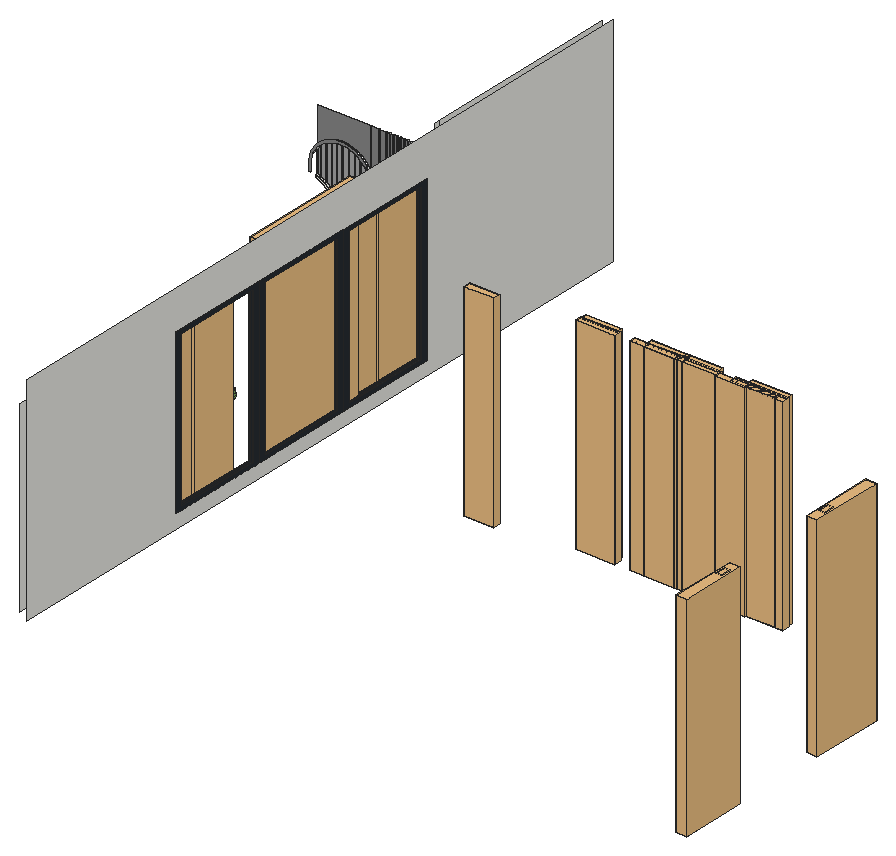
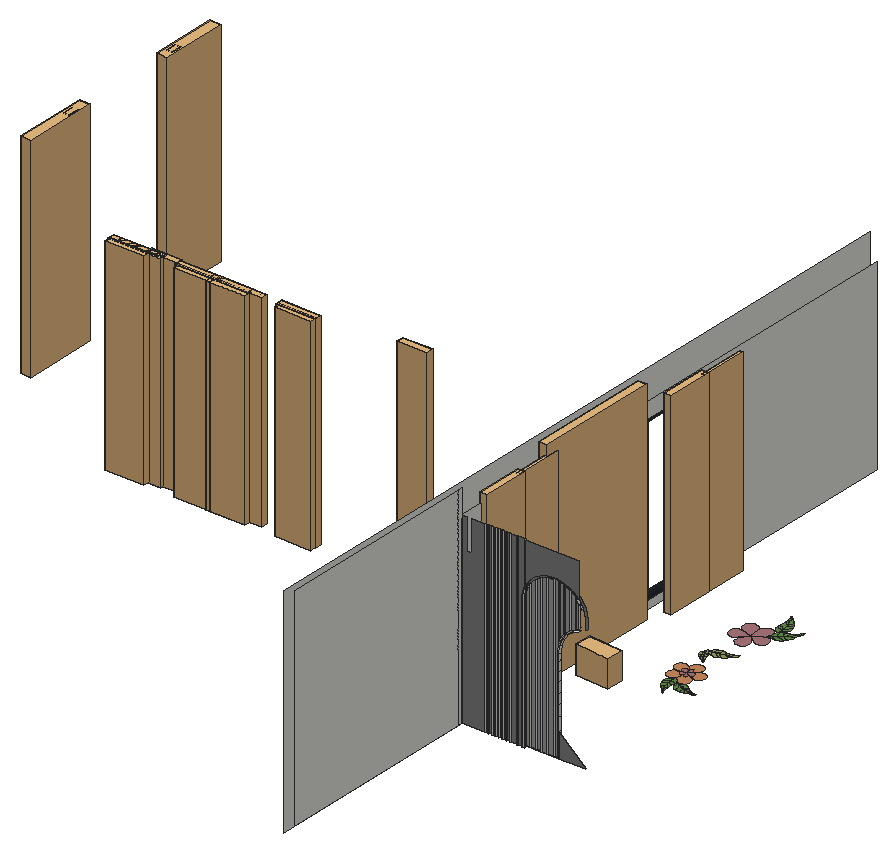
# SketchUp Ruby script. Lengths in inches.
U = 1.inch
M = Sketchup.active_model
def pt(a) = Geom::Point3d.new(a.map { |v| v * U })
def face(e, loops, mat)
  f = e.add_face(loops[0].map { |a| pt(a) })
  loops[1..].each { |l| e.add_face(l.map { |a| pt(a) }).erase! }
  f.material = f.back_material = mat if mat
  f
end
# faces: each face lists its corners as indices into pts; further lists are holes
def faces(e, pts, list, mat = nil) = list.each { |f| face(e, (f[0].is_a?(Array) ? f : [f]).map { |l| l.map { |i| pts[i] } }, mat) }
# xy, xz, yz: faces in a plane at the given z, y or x. An outline is a flat list of corners, or four numbers for a rectangle; further outlines are holes
def ring(l) = l.size == 4 ? [[l[0], l[1]], [l[2], l[1]], [l[2], l[3]], [l[0], l[3]]] : l.each_slice(2).to_a
def flat(e, list, mat, &to3) = list.each { |f| face(e, (f[0].is_a?(Array) ? f : [f]).map { |l| ring(l).map { |u, v| to3.(u, v) } }, mat) }
def xy(e, z, list, mat = nil) = flat(e, list, mat) { |x, y| [x, y, z] }
def xz(e, y, list, mat = nil) = flat(e, list, mat) { |x, z| [x, y, z] }
def yz(e, x, list, mat = nil) = flat(e, list, mat) { |y, z| [x, y, z] }
def lines(e, pts, list) = list.each { |a, b| e.add_line(pt(pts[a]), pt(pts[b])) }
# prism: a flat outline (further loops are holes) pulled along v
def prism(e, loops, v, mat = nil)
  f = face(e, loops, mat); d = Geom::Vector3d.new(v.map { |x| x * U })
  f.pushpull(f.normal.samedirection?(d) ? d.length : -d.length)
end
def box(e, o, s, mat = nil) = prism(e, [[o, [o[0] + s[0], o[1], o[2]], [o[0] + s[0], o[1] + s[1], o[2]], [o[0], o[1] + s[1], o[2]]]], [0, 0, s[2]], mat)
def at(x, y, z, deg = 0) = Geom::Transformation.translation(pt([x, y, z])) * Geom::Transformation.rotation(ORIGIN, Z_AXIS, deg.degrees)
def axes(o, x, y, z) = Geom::Transformation.new([*x, 0, *y, 0, *z, 0, *pt(o).to_a, 1])
def part(name) = M.definitions.add(name)
# library, detail: a bought-in or finely detailed component or shape, given as its bounding box
def library(name, o, s) = part(name).tap { |d| box(d.entities, o, s) }
def detail(e, o, s) = box(e.add_group.entities, o, s)
def put(e, d, t, mat = nil) = e.add_instance(d, t).tap { |i| i.material = mat if mat }
def group(e, t, mat = nil) = e.add_group.tap { |g| g.transformation = t; g.material = mat if mat }.entities
root = M.entities
M.materials.add("Carpet_Frieze_Low").color = [170, 156, 146]
M.materials.add("Carpet_Loop_Low").color = [201, 172, 127]
M.materials["Carpet_Loop_Low"].alpha = 0.3
M.materials.add("Material~3").color = [0, 0, 0]
M.materials.add("Wine2").color = [0, 0, 0]
M.materials["Wine2"].alpha = 0
M.materials.add("[0130_Gainsboro]").color = [39, 45, 50]
M.materials.add("[0132_LightGray]").color = [135, 135, 135]
M.materials.add("[0132_LightGray]1").color = [169, 169, 169]
M.materials.add("[Color_001]1").color = [196, 196, 196]
M.materials["[Color_001]1"].alpha = 0.97
M.materials.add("[Fabric Linen]").color = [168, 116, 117]
M.materials.add("[Granite Tile]").color = [201, 139, 95]
M.materials.add("[Vegetation Blur 01]").color = [168, 117, 122]
M.materials.add("[Vegetation Grass Artificial]").color = [98, 140, 74]
M.materials.add("[Vegetation Grass]").color = [144, 160, 91]
c1 = part("Group\#33")
xy(c1.entities,0,[[3.16,0,2.86,0.82,1.26,2.77,0,5.57,0.11,6.86,0.4375,6.76,0.52,6.68,0.63,6.49,1.02,6.09,1.86,5.44,2.36,5.07,2.77,4.84,3.39,4.72,3.7,4.65,4.07,4.27,3.85,2.85,3.75,2.45],[3.16,0,3.75,2.45,4.12,2.5,4.33,2.64,4.83,2.9,6,3.45,6.93,3.96,7.42,4.13,7.62,4.24,7.93,4.17,7.65,3.64,5.62,1.44],[3.75,2.45,3.85,2.85,4.07,4.27,4.28,5.69,4.62,5.72,4.99,5.91,5.7,6.28,6.96,7,8.1,7.62,9.16,8.86,9.08,6.35,8.01,4.32,7.93,4.17,7.62,4.24,7.42,4.13,6.93,3.96,6,3.45,4.83,2.9,4.33,2.64,4.12,2.5],[4.07,4.27,3.7,4.65,3.39,4.72,2.77,4.84,2.36,5.07,1.86,5.44,1.02,6.09,0.63,6.49,0.52,6.68,0.4375,6.76,0.11,6.86,0.14,7.22,0.28,8.87,0.86,10.33,1.05,9.89,1.35,9.64,1.86,9.3125,2.43,9.02,2.94,8.61,3.51,7.66,3.92,7.21,4.43,6.89,4.28,5.69],[4.28,5.69,4.43,6.89,4.58,8.08,4.59,8.84,4.91,8.96,5.15,9.24,5.74,9.79,6.26,10.125,6.8,10.3125,7.37,10.58,7.8,10.9,8.23,11.24,8.64,11.89,9.16,8.86,8.1,7.62,6.96,7,5.7,6.28,4.99,5.91,4.62,5.72],
  [4.43,6.89,3.92,7.21,3.51,7.66,2.94,8.61,2.43,9.02,1.86,9.3125,1.35,9.64,1.05,9.89,0.86,10.33,1.44,11.8,1.87,13.11,2.28,13.24,2.5,13.125,2.83,12.88,3.0625,12.74,3.16,12.51,3.3,12.2,3.96,11.625,4.28,11.32,4.5,11.15,4.6,11.16,4.61,10.45,4.59,8.84,4.58,8.08],[4.59,8.84,4.61,10.45,4.6,11.16,4.58,12.86,4.66,13.19,4.88,13.24,5.22,13.32,5.85,13.71,6.06,14.02,6.21,14.38,6.39,14.7,6.78,15.17,7.14,14.6,8.64,11.89,8.23,11.24,7.8,10.9,7.37,10.58,6.8,10.3125,6.26,10.125,5.74,9.79,5.15,9.24,4.91,8.96],[4.5,11.15,4.28,11.32,3.96,11.625,3.3,12.2,3.16,12.51,3.0625,12.74,2.83,12.88,2.5,13.125,2.28,13.24,1.87,13.11,2.29,14.41,2.4,16.15,3.04,16.01,3.53,15.76,4.54,15.27,4.58,12.86,4.6,11.16],[4.58,12.86,4.54,15.27,3.82,17.41,3.98,17.35,4.0625,17.43,4.29,17.71,4.85,18.28,6.78,15.17,6.39,14.7,6.21,14.38,6.06,14.02,5.85,13.71,5.22,13.32,4.88,13.24,4.66,13.19],[4.54,15.27,3.53,15.76,3.04,16.01,2.4,16.15,2.51,17.89,2.36,19.5,3.27,19.22,3.62,18.5625,3.82,17.41],
  [3.98,17.35,3.82,17.41,3.62,18.5625,3.27,19.22,2.97,19.94,2.74,20.53,2.73,21.38,3.15,20.92,4.15,19.41,4.85,18.28,4.29,17.71,4.0625,17.43],[3.27,19.22,2.36,19.5,2.21,21.11,2.74,20.53,2.97,19.94],[2.74,20.53,2.21,21.11,2.22,21.31,2.1875,21.5,2.16,21.66,2.15,21.73,2.13,21.81,2.18,21.79,2.45,21.6,2.6,21.53,2.73,21.38]])
c2 = part("Group\#34")
xy(c2.entities,0,[[9.92,0,2.48,3.46,1.45,4.25,0.66,5.28,0.17,6.47,0,7.76,0.17,9.04,0.66,10.24,1.45,11.26,2.48,12.05,3.68,12.55,4.96,12.72,6.24,12.55,7.44,12.05,8.47,11.26,9.26,10.24,9.75,9.04,9.92,7.76]])
c3 = part("Group\#36")
xy(c3.entities,0,[[9.92,0,2.48,3.46,1.45,4.25,0.66,5.28,0.17,6.47,0,7.76,0.17,9.04,0.66,10.24,1.45,11.26,2.48,12.05,3.68,12.55,4.96,12.72,6.24,12.55,7.44,12.05,8.47,11.26,9.26,10.24,9.75,9.04,9.92,7.76]])
c4 = part("Group\#38")
put(c4.entities,c1,at(-0.96,4.16,0,-54.9))
put(c4.entities,c1,at(0.46,7.11,0,4.699))
c5 = part("Group\#60")
g1 = group(c5.entities,at(9.35,11.87,0))
xy(g1,0,[[2.08,-11.87,1.91,-11.81,1.82,-11.79,1.73,-11.73,1.59,-11.28,1.96,-11.51,1.99,-11.61,2.03,-11.71,2.1,-11.85,2.1,-11.87],[1.73,-11.73,1.4375,-11.55,0.68,-10.9,0.14,-10.4,0.36,-10.02,0.43,-9.83,0.47,-9.78,0.56,-9.79,0.84,-10.37,1.12,-10.67,1.38,-11,1.59,-11.28],[1.96,-11.51,1.59,-11.28,1.38,-11,1.12,-10.67,1.64,-10.68],[1.64,-10.68,1.12,-10.67,0.84,-10.37,0.56,-9.79,-0.14,-8.76,0.47,-8.87,0.76,-8.93,1.125,-8.91,1.32,-9.85],[0.14,-10.4,-1.34,-9.04,-1.2,-8.73,-1.16,-8.54,-1.13,-8.32,-1.0625,-8.13,-0.79,-7.83,-0.62,-7.74,-0.51,-7.68,-0.52,-7.49,-0.14,-8.76,0.56,-9.79,0.47,-9.78,0.43,-9.83,0.36,-10.02],
  [-1.34,-9.04,-1.62,-8.79,-2.81,-7.58,-2.69,-7.17,-2.52,-6.93,-2.33,-6.69,-2.07,-6.47,-1.81,-6.29,-1.59,-6.04,-1.36,-5.66,-1.27,-5.47,-1.12,-5.36,-0.89,-6.22,-0.78,-6.59,-0.52,-7.49,-0.51,-7.68,-0.62,-7.74,-0.79,-7.83,-1.0625,-8.13,-1.13,-8.32,-1.16,-8.54,-1.2,-8.73],[0.76,-8.93,0.47,-8.87,-0.14,-8.76,-0.52,-7.49,-0.78,-6.59,-0.73,-6.57,-0.59,-6.63,-0.37,-6.74,0.0625,-6.95,0.18,-7.09,0.27,-7.2,0.41,-7.24,0.62,-7.32,0.75,-7.35,0.96,-7.22,0.92,-7.97,1.125,-8.91],[-2.81,-7.58,-3.54,-6.05,-3.16,-5.24,-2.65,-4.74,-2.09,-4.17,-1.77,-3.87,-1.6,-3.71,-1.42,-3.65,-1.33,-4.31,-1.23,-4.96,-1.12,-5.36,-1.27,-5.47,-1.36,-5.66,-1.59,-6.04,-1.81,-6.29,-2.07,-6.47,-2.33,-6.69,-2.52,-6.93,-2.69,-7.17],[0.75,-7.35,0.62,-7.32,0.41,-7.24,0.27,-7.2,0.18,-7.09,0.0625,-6.95,-0.37,-6.74,-0.59,-6.63,-0.73,-6.57,-0.78,-6.59,-0.89,-6.22,-1.12,-5.36,-1.23,-4.96,-1.33,-4.31,-1.01,-4.4,-0.72,-4.58,-0.28,-5,0.05,-5.14,0.4,-5.21,0.71,-5.31,0.91,-5.4,1.08,-5.6,0.99,-6.46,0.96,-7.22],[-3.54,-6.05,-3.87,-4.71,-3.6,-3.47,-3.58,-3.39,-3.41,-3.375,-3.32,-3.29,-3.08,-3.13,-2.67,-2.72,-2.13,-2.25,-1.9,-2.04,-1.8125,-1.9375,-1.625,-1.85,-1.62,-2.08,-1.52,-2.86,-1.42,-3.65,-1.6,-3.71,-1.77,-3.87,-2.09,-4.17,-2.65,-4.74,-3.16,-5.24],
  [1.08,-5.6,0.91,-5.4,0.71,-5.31,0.4,-5.21,0.05,-5.14,-0.28,-5,-0.72,-4.58,-1.01,-4.4,-1.33,-4.31,-1.42,-3.65,-1.52,-2.86,-1.27,-3.01,-1.09,-3,-0.75,-2.98,-0.5,-3.04,-0.18,-3.16,0.36,-3.375,0.63,-3.53,0.72,-3.61,0.77,-3.64,0.96,-3.65,1,-3.84,1.17,-4.74],[0.96,-3.65,0.77,-3.64,0.72,-3.61,0.63,-3.53,0.36,-3.375,-0.18,-3.16,-0.5,-3.04,-0.75,-2.98,-1.09,-3,-1.27,-3.01,-1.52,-2.86,-1.62,-2.08,-1.625,-1.85,-1.67,-0.47,-1.39,-0.86,-0.26,-1.66,0.83,-2.95],[-3.58,-3.39,-3.51,-3.0625,-2.76,-1.6,-1.67,-0.47,-1.625,-1.85,-1.8125,-1.9375,-1.9,-2.04,-2.13,-2.25,-2.67,-2.72,-3.08,-3.13,-3.32,-3.29,-3.41,-3.375]])
put(c5.entities,c1,axes([8.26,10.79,0],[-0.18907,0.36013,0],[-0.36013,-0.18907,0],[0,0,1]))
c6 = library("Throw pillow",[0,0,0],[9.42,19.46,15.55])
c7 = library("Group\#2",[0,0,0],[27.01,4.84,111.86])
c8 = library("3DGeom~1_Defintion\#7",[122.66,-414.5625,-71.91],[799.29,1000,104.01])
c9 = part("Group9\#3")
put(c9.entities,c8,axes([11.875,801.95,874.35],[0,-1.454,0],[0,0,2.10433],[-1.32595,0,0]),"Material~3")
c10 = part("Group8\#3")
put(c10.entities,c9,at(0,0,0))
c11 = part("Framed glazing panel")
xy(c11.entities,0,[[0,-0.98,43.07,0],[0,0,43.07,1.4]],"[0130_Gainsboro]")
xy(c11.entities,0.3,[[0.3,-1.43,42.77,-0.98]],"[0130_Gainsboro]")
xy(c11.entities,2.95,[[2.95,-1.43,40.12,-0.63],[2.95,-0.63,40.12,0],[2.95,0,40.12,0.64],[2.95,0.64,40.12,1.4]],"[0130_Gainsboro]")
xy(c11.entities,3.54,[[3.54,-0.63,39.53,0],[3.54,0,39.53,0.64]],"[0130_Gainsboro]")
xy(c11.entities,111.8125,[[3.54,-0.63,39.53,0],[3.54,0,39.53,0.64]],"[0130_Gainsboro]")
xy(c11.entities,112.4,[[2.95,-1.43,40.12,-0.63],[2.95,-0.63,40.12,0],[2.95,0,40.12,0.64],[2.95,0.64,40.12,1.4]],"[0130_Gainsboro]")
xy(c11.entities,115.05,[[0.3,-1.43,42.77,-0.98]],"[0130_Gainsboro]")
xy(c11.entities,115.35,[[0,-0.98,43.07,0],[0,0,43.07,1.4]],"[0130_Gainsboro]")
xz(c11.entities,-1.43,[[[0.3,0.3,42.77,115.05],[2.95,2.95,40.12,112.4]]],"[0130_Gainsboro]")
xz(c11.entities,-0.98,[[[0,0,43.07,115.35],[0.3,0.3,42.77,115.05]]],"[0130_Gainsboro]")
xz(c11.entities,-0.63,[[[2.95,2.95,40.12,112.4],[3.54,3.54,39.53,111.8125]]],"[0130_Gainsboro]")
xz(c11.entities,0,[[3.54,3.54,39.53,111.8125]],"Wine2")
xz(c11.entities,0,[[[0,0,43.07,115.35],[2.95,2.95,40.12,112.4]],[[2.95,2.95,40.12,112.4],[3.54,3.54,39.53,111.8125]]],"[0130_Gainsboro]")
xz(c11.entities,0.64,[[[2.95,2.95,40.12,112.4],[3.54,3.54,39.53,111.8125]]],"[0130_Gainsboro]")
xz(c11.entities,1.4,[[[0,0,43.07,115.35],[2.95,2.95,40.12,112.4]]],"[0130_Gainsboro]")
yz(c11.entities,0,[[-0.98,0,0,115.35],[0,0,1.4,115.35]],"[0130_Gainsboro]")
yz(c11.entities,0.3,[[-1.43,0.3,-0.98,115.05]],"[0130_Gainsboro]")
yz(c11.entities,2.95,[[-1.43,2.95,-0.63,112.4],[-0.63,2.95,0,112.4],[0,2.95,0.64,112.4],[0.64,2.95,1.4,112.4]],"[0130_Gainsboro]")
yz(c11.entities,3.54,[[-0.63,3.54,0,111.8125],[0,3.54,0.64,111.8125]],"[0130_Gainsboro]")
yz(c11.entities,39.53,[[-0.63,3.54,0,111.8125],[0,3.54,0.64,111.8125]],"[0130_Gainsboro]")
yz(c11.entities,40.12,[[-1.43,2.95,-0.63,112.4],[-0.63,2.95,0,112.4],[0,2.95,0.64,112.4],[0.64,2.95,1.4,112.4]],"[0130_Gainsboro]")
yz(c11.entities,42.77,[[-1.43,0.3,-0.98,115.05]],"[0130_Gainsboro]")
yz(c11.entities,43.07,[[-0.98,0,0,115.35],[0,0,1.4,115.35]],"[0130_Gainsboro]")
c12 = part("Glazed panel assembly")
put(c12.entities,c11,axes([90.57,1.43,0],[1.05148,0,0],[0,1,0],[0,0,1]))
put(c12.entities,c11,axes([0,1.43,0],[1.05148,0,0],[0,1,0],[0,0,1]))
put(c12.entities,c11,axes([45.29,1.43,0],[1.05148,0,0],[0,1,0],[0,0,1]))
c13 = part("Curtain panel")
p = [[5.51,1.25,0],[5.9,0.93,0],[4.95,2.09,0],[5.1875,1.64,0],[6.35,0.69,0],[6.83,0.55,0],
  [7.33,0.5,0],[7.84,0.55,0],[8.32,0.69,0],[8.77,0.93,0],[9.16,1.25,0],[9.48,1.64,0],
  [9.72,2.09,0],[10,2.61,0],[10.375,3.0625,0],[10.83,3.4375,0],[17.64,0.16,0],[18.27,0.1,0],
  [11.35,3.71,0],[11.92,3.89,0],[12.51,3.94,0],[13.09,3.89,0],[20.56,1.04,0],[20.96,1.53,0],
  [13.66,3.71,0],[14.18,3.4375,0],[14.64,3.0625,0],[15.01,2.61,0],[15.29,2.09,0],[15.59,1.53,0],
  [15.99,1.04,0],[16.48,0.64,0],[17.04,0.34,0],[18.9,0.16,0],[19.51,0.34,0],[20.07,0.64,0],
  [21.26,2.09,0],[21.56,2.64,0],[21.96,3.13,0],[22.45,3.53,0],[23,3.83,0],[23.61,4.01,0],
  [24.24,4.08,0],[24.25,3.98,0]]
lines(c13.entities,p,[[0,1],[2,3],[3,0],[1,4],[4,5],[5,6],[6,7],[7,8],[8,9],[9,10],[10,11],[11,12],
  [12,13],[13,14],[14,15],[16,17],[15,18],[18,19],[19,20],[20,21],[22,23],[21,24],[24,25],[25,26],
  [26,27],[27,28],[28,29],[29,30],[30,31],[31,32],[32,16],[17,33],[33,34],[34,35],[35,22],[23,36],
  [36,37],[37,38],[38,39],[39,40],[40,41],[41,42],[42,43]])
detail(c13.entities,[0.85,0,0],[23.4,3.98,78.74])
c14 = part("Group\#57")
put(c14.entities,c13,axes([-0.76,0,0],[0.8979,0,0],[0,1,0],[0,0,1]),"Carpet_Frieze_Low")
put(c14.entities,c13,axes([37.23,0,0],[0.9782,0,0],[0,1,0],[0,0,1]),"Carpet_Frieze_Low")
c15 = library("Group14\#3",[-63.24,-641.87,2.3125],[92.6,96.43,2109.15])
c16 = library("3DGeom~5_Defintion\#6",[-129.21,-457.45,-50.66],[372.46,1000,95.96])
c17 = part("Group15\#3")
put(c17.entities,c16,axes([-25.11,-678.68,967.09],[0,-1.68483,0],[0,0,2.10997],[-1.81292,0,0]),"Material~3")
c18 = part("Group13\#3")
put(c18.entities,c15,at(0,0,0),"[Color_001]1")
put(c18.entities,c17,at(0,0,0))
c19 = library("Group11\#3",[-63.24,494.46,2.3125],[92.6,100.74,2109.15])
c20 = library("3DGeom~3_Defintion\#7",[-166.03,-457.45,-50.66],[409.15,1000,95.96])
c21 = part("Group12\#3")
put(c21.entities,c20,axes([-25.11,656.6,967.09],[0,1.68483,0],[0,0,2.10997],[-1.81292,0,0]),"Material~3")
c22 = part("Group10\#3")
put(c22.entities,c19,at(0,0,0),"[Color_001]1")
put(c22.entities,c21,at(0,0,0))
xy(root,4.42,[[237.73,293.53,256.18,293.53,256.18,294.66,255.74,294.66,255.74,294.91,255.66,294.91,255.66,294.66,253.09,294.66,253.09,294.91,252.91,294.91,252.91,294.66,249.79,294.66,249.79,294.91,249.64,294.91,249.64,294.66,246.8,294.66,246.8,294.91,246.67,294.91,246.67,294.66,243.31,294.66,243.31,294.91,243.24,294.91,243.24,294.66,239.66,294.66,239.66,294.91,239.57,294.91,239.57,294.41,237.73,294.41]])
xy(root,7.42,[[291.63,105.89,295.1875,285.58]])
xz(root,105.89,[[291.63,7.42,295.1875,100.73]])
xz(root,285.58,[[291.63,7.42,295.1875,100.73]])
xz(root,293.53,[[237.73,3.125,257.75,3.125,257.75,78.24,257.7,79.04,257.62,79.84,257.5,80.63,257.35,81.41,257.16,82.19,256.94,82.96,256.69,83.72,256.41,84.47,256.09,85.2,255.74,85.92,255.36,86.63,254.95,87.32,254.51,87.98,254.05,88.63,253.55,89.26,253.03,89.87,252.48,90.45,251.91,91.01,251.3125,91.55,250.69,92.05,250.06,92.53,249.4,92.99,248.72,93.41,248.02,93.8,247.31,94.16,246.58,94.5,245.84,94.8,245.08,95.0625,244.32,95.3,243.54,95.5,242.76,95.67,241.97,95.8,241.18,95.9,240.38,95.97,239.58,96,238.78,95.99,237.98,95.95,237.1875,95.88,236.39,95.77,235.61,95.63,234.83,95.45,234.05,95.24,233.29,95,232.54,94.73,231.8,94.42,231.08,94.08,230.37,93.71,229.68,93.31,229,92.875,228.35,92.42,227.71,91.93,227.1,91.41,226.51,90.875,225.94,90.31,225.4,89.72,222.51,85.27,221.75,82.74,221.03,80.29,221.03,74.86,221.75,74.76,222.32,74.6875,222.32,80.11,222.99,82.375,223.69,84.72,226.39,88.86,227.05,89.43,230.15,92.0625,233.34,93.47,234.67,94.0625,236.33,94.28,239.57,94.69,243.24,94.09,244.44,93.9,246.67,92.83,248.89,91.75,249.64,91.08,252.54,88.43,252.91,87.83,255.1,84.21,256.22,79.91,256.35,79.43,256.18,74.28,256.18,4.42,237.73,4.42]],"[0132_LightGray]")
xz(root,294.41,[[237.73,4.42,239.57,4.42,239.57,94.69,236.47,94.29,236.47,64.13,237.16,62.46,237.73,58.125]],"[0132_LightGray]1")
xz(root,294.47,[[257.75,3.125,260.26,3.125,260.26,109.39,255.93,109.39,255.93,85.52,256.09,85.2,256.41,84.47,256.69,83.72,256.94,82.96,257.16,82.19,257.35,81.41,257.5,80.63,257.62,79.84,257.7,79.04,257.75,78.24,257.76,77.44,257.75,76.89],[260.79,3.125,264.44,109.39],[264.79,3.125,266.48,109.39],[266.83,3.125,268.52,109.39],[268.86,3.125,270.55,109.39],
  [270.9,3.125,272.59,109.39],[272.94,3.125,274.63,109.39],[274.98,3.125,276.67,109.39],[277.02,3.125,278.7,109.39]],"[0132_LightGray]")
xz(root,294.66,[[239.66,4.42,243.24,4.42,243.24,94.09,239.66,94.68],[243.31,4.42,246.67,4.42,246.67,92.83,244.44,93.9,243.31,94.08],[246.8,4.42,249.64,4.42,249.64,91.08,248.89,91.75,246.8,92.76],[249.79,4.42,252.91,4.42,252.91,87.83,252.54,88.43,249.79,90.9375],[253.09,4.42,255.66,4.42,255.66,82.06,255.1,84.21,253.09,87.52],
  [255.74,4.42,256.18,4.42,256.18,74.28,256.35,79.43,256.22,79.91,255.74,81.76],[236.33,64.45,236.33,94.28,234.67,94.0625,233.56,93.57,233.56,69.01,235.49,66.49],[233.34,69.3,233.34,93.47,230.375,92.16,230.375,71.84,232.83,69.96],[230.15,72.02,230.15,92.0625,227.17,89.53,227.17,73.53,229.36,72.62],[227.05,73.58,227.05,89.43,226.39,88.86,225.18,87.01,225.18,74.3125,225.32,74.29,225.4,74.26]],"[0132_LightGray]1")
xz(root,294.91,[[255.93,3.125,257.75,3.125,257.75,78.24,257.7,79.04,257.62,79.84,257.5,80.63,257.35,81.41,257.16,82.19,256.94,82.96,256.69,83.72,256.41,84.47,256.09,85.2,255.93,85.52],[264.44,3.125,264.79,109.39],[266.48,3.125,266.83,109.39],[268.52,3.125,268.86,109.39],[239.57,4.42,239.66,4.42,239.66,94.68,239.57,94.69],
  [243.24,4.42,243.31,4.42,243.31,94.08,243.24,94.09],[246.67,4.42,246.8,4.42,246.8,92.76,246.67,92.83],[249.64,4.42,249.79,4.42,249.79,90.9375,249.64,91.08],[252.91,4.42,253.09,4.42,253.09,87.52,252.91,87.83],[255.66,4.42,255.74,4.42,255.74,81.76,255.66,82.06],
  [236.47,64.13,236.47,94.29,236.33,94.28,236.33,64.45],[233.56,69.01,233.56,93.57,233.34,93.47,233.34,69.3],[230.375,71.84,230.375,92.16,230.15,92.0625,230.15,72.02],[227.17,73.53,227.17,89.53,227.05,89.43,227.05,73.58],[225.18,74.3125,225.18,87.01,225.04,86.79,225.04,74.33],
  [257.75,76.89,257.76,77.44,257.75,78.24]])
xz(root,294.91,[[260.26,3.125,260.79,109.39],[270.55,3.125,270.9,109.39],[272.59,3.125,272.94,109.39],[274.63,3.125,274.98,109.39],[276.67,3.125,277.02,109.39],
  [278.7,3.125,291.63,3.125,291.63,109.39,289,109.39,289,91.83,286.12,91.83,286.12,109.39,278.7,109.39],[220.99,4.38,236.48,4.38,236.48,17.84],[255.93,85.52,255.93,109.39,225.4,109.39,225.4,89.72,225.94,90.31,226.51,90.875,227.1,91.41,227.71,91.93,228.35,92.42,229,92.875,229.68,93.31,230.37,93.71,231.08,94.08,231.8,94.42,232.54,94.73,233.29,95,234.05,95.24,234.83,95.45,235.61,95.63,236.39,95.77,237.1875,95.88,237.98,95.95,238.78,95.99,239.58,96,240.38,95.97,241.18,95.9,241.97,95.8,242.76,95.67,243.54,95.5,244.32,95.3,245.08,95.0625,245.84,94.8,246.58,94.5,247.31,94.16,248.02,93.8,248.72,93.41,249.4,92.99,250.06,92.53,250.69,92.05,251.3125,91.55,251.91,91.01,252.48,90.45,253.03,89.87,253.55,89.26,254.05,88.63,254.51,87.98,254.95,87.32,255.36,86.63,255.74,85.92]],"[0132_LightGray]")
yz(root,225.04,[[294.66,74.33,294.91,86.79]])
yz(root,225.18,[[294.66,74.3125,294.91,87.01]])
yz(root,227.05,[[294.66,73.58,294.91,89.43]])
yz(root,227.17,[[294.66,73.53,294.91,89.53]])
yz(root,230.15,[[294.66,72.02,294.91,92.0625]])
yz(root,230.375,[[294.66,71.84,294.91,92.16]])
yz(root,233.34,[[294.66,69.3,294.91,93.47]])
yz(root,233.56,[[294.66,69.01,294.91,93.57]])
yz(root,236.33,[[294.66,64.45,294.91,94.28]])
yz(root,236.47,[[294.41,64.13,294.91,94.29]])
yz(root,236.48,[[293.53,4.38,294.91,17.84],[293.53,17.84,294.91,25.84],[293.53,25.84,294.91,31.64],[293.53,31.64,294.91,37.31],[293.53,37.31,294.91,43.35],
  [293.53,43.35,294.91,48.5],[293.53,48.5,294.91,54.0625],[293.53,54.0625,294.91,58.04]])
yz(root,237.73,[[293.53,4.42,294.41,58.125]])
yz(root,239.57,[[294.41,4.42,294.91,94.69]])
yz(root,239.66,[[294.66,4.42,294.91,94.68]])
yz(root,243.24,[[294.66,4.42,294.91,94.09]])
yz(root,243.31,[[294.66,4.42,294.91,94.08]])
yz(root,246.67,[[294.66,4.42,294.91,92.83]])
yz(root,246.8,[[294.66,4.42,294.91,92.76]])
yz(root,249.64,[[294.66,4.42,294.91,91.08]])
yz(root,249.79,[[294.66,4.42,294.91,90.9375]])
yz(root,252.91,[[294.66,4.42,294.91,87.83]])
yz(root,253.09,[[294.66,4.42,294.91,87.52]])
yz(root,255.66,[[294.66,4.42,294.91,82.06]])
yz(root,255.74,[[294.66,4.42,294.91,81.76]])
yz(root,255.93,[[294.47,85.52,294.91,109.39]])
yz(root,256.18,[[293.53,4.42,294.66,74.28]])
yz(root,257.75,[[293.53,3.125,294.47,76.89],[294.47,3.125,294.91,76.89],[293.53,76.89,294.91,78.24]])
yz(root,260.26,[[294.47,3.125,294.91,109.39]])
yz(root,260.79,[[294.47,3.125,294.91,109.39]])
yz(root,264.44,[[294.47,3.125,294.91,109.39]])
yz(root,264.79,[[294.47,3.125,294.91,109.39]])
yz(root,266.48,[[294.47,3.125,294.91,109.39]])
yz(root,266.83,[[294.47,3.125,294.91,109.39]])
yz(root,268.52,[[294.47,3.125,294.91,109.39]])
yz(root,268.86,[[294.47,3.125,294.91,109.39]])
yz(root,270.55,[[294.47,3.125,294.91,109.39]])
yz(root,270.9,[[294.47,3.125,294.91,109.39]])
yz(root,272.59,[[294.47,3.125,294.91,109.39]])
yz(root,272.94,[[294.47,3.125,294.91,109.39]])
yz(root,274.63,[[294.47,3.125,294.91,109.39]])
yz(root,274.98,[[294.47,3.125,294.91,109.39]])
yz(root,276.67,[[294.47,3.125,294.91,109.39]])
yz(root,277.02,[[294.47,3.125,294.91,109.39]])
yz(root,278.7,[[294.47,3.125,294.91,109.39]])
yz(root,291.63,[[[0,3.125,294.91,109.39],[105.89,7.42,285.58,100.73]],[294.91,3.125,298.46,123.125],[298.46,3.125,414.13,123.125]])
yz(root,295.1875,[[[0,0,417.6875,123.125],[105.89,7.42,285.58,100.73]]])
p = [[235.94,294.91,62.13],[236.48,294.91,58.04],[236.48,293.53,58.04],[235.94,293.53,62.13],[237.73,293.53,58.125],[237.73,294.41,58.125],
  [237.16,294.41,62.46],[237.16,293.53,62.46],[234.39,294.91,65.86],[234.39,293.53,65.86],[236.47,294.41,64.13],[236.47,294.91,64.13],
  [236.33,294.91,64.45],[236.33,294.66,64.45],[236.33,293.53,64.45],[235.49,294.66,66.49],[235.49,293.53,66.49],[231.93,294.91,69.07],
  [231.93,293.53,69.07],[233.56,294.66,69.01],[233.56,294.91,69.01],[233.34,294.91,69.3],[233.34,294.66,69.3],[233.34,293.53,69.3],
  [228.73,294.91,71.53],[228.73,293.53,71.53],[232.83,294.66,69.96],[232.83,293.53,69.96],[230.375,294.66,71.84],[230.375,294.91,71.84],
  [230.15,294.91,72.02],[230.15,294.66,72.02],[230.15,293.53,72.02],[225,294.91,73.07],[225,293.53,73.07],[229.36,294.66,72.62],
  [229.36,293.53,72.62],[227.17,294.66,73.53],[227.17,294.91,73.53],[227.05,294.91,73.58],[227.05,294.66,73.58],[227.05,293.53,73.58],
  [225.4,294.66,74.26],[225.4,293.53,74.26],[225.32,293.53,74.29],[225.32,294.66,74.29],[225.18,294.66,74.3125],[225.18,294.91,74.3125],
  [225.04,294.91,74.33],[225.04,294.66,74.33],[225.04,293.53,74.33],[256.35,293.53,79.43],[256.35,294.66,79.43],[256.18,294.66,74.28],
  [256.18,293.53,74.28],[257.76,294.91,77.44],[257.75,294.91,76.89],[257.75,294.47,76.89],[257.76,294.47,77.44],[257.75,294.91,78.24],
  [257.75,294.47,78.24],[257.75,293.53,78.24],[257.7,294.47,79.04],[257.7,293.53,79.04],[257.7,294.91,79.04],[257.62,294.47,79.84],
  [257.62,293.53,79.84],[257.62,294.91,79.84],[256.22,293.53,79.91],[256.22,294.66,79.91],[257.5,294.47,80.63],[257.5,293.53,80.63],
  [257.5,294.91,80.63],[255.66,294.91,82.06],[255.74,294.91,81.76],[255.74,294.66,81.76],[255.66,293.53,82.06],[255.66,294.66,82.06],
  [257.35,294.47,81.41],[257.35,293.53,81.41],[257.35,294.91,81.41],[257.16,294.47,82.19],[257.16,293.53,82.19],[257.16,294.91,82.19],
  [255.1,293.53,84.21],[255.1,294.66,84.21],[256.94,294.47,82.96],[256.94,293.53,82.96],[256.94,294.91,82.96],[256.69,294.47,83.72],
  [256.69,293.53,83.72],[256.69,294.91,83.72],[256.41,294.47,84.47],[256.41,293.53,84.47],[256.41,294.91,84.47],[252.91,294.91,87.83],
  [253.09,294.91,87.52],[253.09,294.66,87.52],[252.91,293.53,87.83],[252.91,294.66,87.83],[256.09,294.47,85.2],[256.09,293.53,85.2],
  [256.09,294.91,85.2],[223.69,293.53,84.72],[223.69,294.66,84.72],[225.04,294.66,86.79],[225.04,293.53,86.79],[255.93,294.91,85.52],
  [255.74,294.91,85.92],[255.74,293.53,85.92],[255.93,294.47,85.52],[255.36,294.91,86.63],[255.36,293.53,86.63],[254.95,294.91,87.32],
  [254.95,293.53,87.32],[225.04,294.91,86.79],[225.18,294.91,87.01],[225.18,294.66,87.01],[226.39,294.66,88.86],[226.39,293.53,88.86],
  [254.51,294.91,87.98],[254.51,293.53,87.98],[536.17,204.67,116.93],[536.17,204.67,0],[536.33,204.95,0],[536.33,204.95,116.93],
  [542.91,203.77,0],[542.91,203.77,116.93],[550.09,203.5,116.93],[550.09,203.5,0],[525.49,203.34,0],[525.49,203.34,116.93],
  [478.85,204.95,0],[478.85,204.95,116.93],[468.01,203.34,0],[468.01,203.34,116.93],[478.69,204.67,116.93],[478.69,204.67,0],
  [492.61,203.5,116.93],[492.61,203.5,0],[485.43,203.77,0],[485.43,203.77,116.93]]
faces(root,p,[[0,1,2,3],[4,5,6,7],[8,0,3,9],[7,6,10,11,12,13,14],[14,13,15,16],[17,8,9,18],[16,15,19,20,21,22,23],[24,17,18,25],
  [23,22,26,27],[27,26,28,29,30,31,32],[33,24,25,34],[32,31,35,36],[36,35,37,38,39,40,41],[41,40,42,43],[44,45,46,47,48,49,50],[43,42,45,44],
  [51,52,53,54],[55,56,57,58],[59,55,58,60],[61,60,62,63],[59,64,62,60],[63,62,65,66],[64,67,65,62],[68,69,52,51],
  [66,65,70,71],[67,72,70,65],[73,74,75,69,68,76,77],[71,70,78,79],[72,80,78,70],[79,78,81,82],[80,83,81,78],[84,85,77,76],
  [82,81,86,87],[83,88,86,81],[87,86,89,90],[88,91,89,86],[90,89,92,93],[91,94,92,89],[95,96,97,85,84,98,99],[93,92,100,101],
  [94,102,100,92],[103,104,105,106],[107,108,109,101,100,110],[102,107,110,100],[108,111,112,109],[111,113,114,112],[115,116,117,118,119,106,105],[113,120,121,114]])
lines(root,p,[[122,123],[124,125],[126,127],[128,129],[130,131],[132,133],[134,135],[136,137],[138,139],[140,141]])
g2 = group(root,at(249.21,165.14,3.61),"[Vegetation Blur 01]")
put(g2,c1,axes([-14.23,-20.27,0],[-0.72896,-0.17769,0],[0.17769,-0.72896,0],[0,0,1.23]),"[Vegetation Grass Artificial]")
put(g2,c2,axes([-1.33,-10.9375,0],[-0.74106,-0.11737,0],[0.11737,-0.74106,0],[0,0,1.23]))
put(g2,c1,axes([-13.53,-17.92,0],[-0.52214,0.53881,0],[-0.53881,-0.52214,0],[0,0,1.23]),"[Vegetation Grass Artificial]")
put(g2,c3,axes([-5.12,-18.64,0],[-0.35916,0.65875,0],[-0.65875,-0.35916,0],[0,0,1.23]))
put(g2,c3,axes([-7.16,-4.8125,0],[-0.15343,-0.73444,0],[0.73444,-0.15343,0],[0,0,1.23]))
put(g2,c3,axes([-13.46,-17.8,0],[0.48228,0.57476,0],[-0.57476,0.48228,0],[0,0,1.23]))
put(g2,c3,axes([-15.3,-8.7,0],[0.66733,-0.34296,0],[0.34296,0.66733,0],[0,0,1.23]))
g3 = group(root,at(246.65,185.23,3.61),"[Vegetation Grass Artificial]")
put(g3,c4,axes([-3.03,17.62,0],[0.25779,0.62546,0],[-0.62546,0.25779,0],[0,0,1.23]))
g4 = group(g3,at(3.77,17.2,0),"[Granite Tile]")
xy(g4,0,[[-7.03,-4.4,-6.57,-4.22,-6.28,-4.01,-6.06,-3.73,-5.91,-3.4,-5.85,-3.05,-5.89,-2.6875,-6.02,-2.35,-6.23,-2.06,-6.51,-1.83,-6.84,-1.6875,-7.2,-1.63,-7.55,-1.67,-7.89,-1.8,-8.18,-2.01,-8.41,-2.29,-8.57,-2.66,-7.92,0.57,-7.5625,1.37,-7.01,2.05,-6.3,2.5625,-5.49,2.875,-4.61,2.97,-3.75,2.83,-2.95,2.47,-2.27,1.92,-1.75,1.21,-1.4375,0.4,-1.35,-0.47,-1.48,-1.34,-1.84,-2.14,-2.39,-2.82,-3.1,-3.34,-3.92,-3.65]])
xy(g4,0,[[-9.02,-4.875,-8.57,-2.66,-8.41,-2.29,-8.18,-2.01,-7.89,-1.8,-7.55,-1.67,-7.2,-1.63,-6.84,-1.6875,-6.51,-1.83,-6.23,-2.06,-6.02,-2.35,-5.89,-2.6875,-5.85,-3.05,-5.91,-3.4,-6.06,-3.73,-6.28,-4.01,-6.57,-4.22,-7.03,-4.4]],"[Fabric Linen]")
g5 = group(g3,at(-6.96,22.43,0),"[Granite Tile]")
xy(g5,0,[[-0.25,-8.97,-3.09,-7.31,-3.73,-6.72,-4.2,-5.98,-4.46,-5.14,-4.49,-4.27,-4.3,-3.41,-3.89,-2.64,-3.29,-1.99,-2.55,-1.53,-1.71,-1.27,-0.84,-1.23,0.01,-1.43,0.79,-1.84,1.43,-2.43,1.9,-3.17,2.16,-4.01,2.19,-4.89,1.9,-8.07,1.88,-7.58,1.77,-7.24,1.58,-6.93,1.32,-6.69,1,-6.52,0.65,-6.44,0.29,-6.46,-0.06,-6.5625,-0.36,-6.75,-0.61,-7.02,-0.78,-7.34,-0.86,-7.6875,-0.84,-8.05,-0.74,-8.39,-0.54,-8.7]])
xy(g5,0,[[1.71,-10.11,-0.25,-8.97,-0.54,-8.7,-0.74,-8.39,-0.84,-8.05,-0.86,-7.6875,-0.78,-7.34,-0.61,-7.02,-0.36,-6.75,-0.06,-6.5625,0.29,-6.46,0.65,-6.44,1,-6.52,1.32,-6.69,1.58,-6.93,1.77,-7.24,1.88,-7.58,1.9,-8.07]],"[Fabric Linen]")
g6 = group(g3,at(-9.75,3.11,0),"[Granite Tile]")
xy(g6,0,[[3.84,-0.3,2.96,-0.24,2.13,0.03,1.4,0.52,0.82,1.17,0.43,1.95,0.25,2.8125,0.3,3.6875,0.58,4.52,1.0625,5.25,3.16,7.67,2.89,7.26,2.77,6.92,2.75,6.56,2.83,6.21,2.99,5.88,3.23,5.61,3.53,5.42,3.87,5.3,4.23,5.28,4.58,5.35,4.9,5.51,5.17,5.75,5.37,6.05,5.48,6.4,5.5,6.76,5.42,7.15,6.77,4.15,6.95,3.29,6.89,2.42,6.62,1.59,6.13,0.85,5.48,0.27,4.7,-0.12]])
xy(g6,0,[[4.23,5.28,3.87,5.3,3.53,5.42,3.23,5.61,2.99,5.88,2.83,6.21,2.75,6.56,2.77,6.92,2.89,7.26,3.16,7.67,4.5,9.21,5.42,7.15,5.5,6.76,5.48,6.4,5.37,6.05,5.17,5.75,4.9,5.51,4.58,5.35]],"[Fabric Linen]")
g7 = group(g3,at(-15.375,13.96,0),"[Granite Tile]")
xy(g7,0,[[4.31,-5.9,3.43,-5.875,2.59,-5.625,1.84,-5.17,1.24,-4.53,0.83,-3.76,0.625,-2.91,0.65,-2.03,0.9,-1.19,1.36,-0.45,1.99,0.16,2.76,0.57,3.62,0.78,4.49,0.75,5.33,0.5,8.25,-0.81,7.78,-0.67,7.42,-0.66,7.07,-0.74,6.76,-0.91,6.5,-1.16,6.31,-1.47,6.2,-1.81,6.19,-2.17,6.28,-2.52,6.45,-2.84,6.7,-3.1,7,-3.29,7.35,-3.39,7.71,-3.4,8.06,-3.32,8.41,-3.125,5.93,-5.28,5.16,-5.7]])
xy(g7,0,[[7.71,-3.4,7.35,-3.39,7,-3.29,6.7,-3.1,6.45,-2.84,6.28,-2.52,6.19,-2.17,6.2,-1.81,6.31,-1.47,6.5,-1.16,6.76,-0.91,7.07,-0.74,7.42,-0.66,7.78,-0.67,8.25,-0.81,10.12,-1.64,8.41,-3.125,8.06,-3.32]],"[Fabric Linen]")
g8 = group(g3,at(2.16,5.24,0),"[Granite Tile]")
xy(g8,0,[[-1.73,1,-2.6,1.09,-3.42,1.41,-4.13,1.93,-4.68,2.61,-6.35,5.34,-6.04,4.96,-5.75,4.75,-5.41,4.62,-5.05,4.58,-4.7,4.63,-4.37,4.78,-4.09,5.01,-3.875,5.3,-3.75,5.63,-3.71,5.99,-3.76,6.35,-3.91,6.68,-4.13,6.96,-4.43,7.17,-4.76,7.3,-5.16,7.34,-1.9,7.71,-1.02,7.62,-0.21,7.3,0.5,6.79,1.05,6.1,1.41,5.3,1.54,4.4375,1.45,3.57,1.13,2.75,0.62,2.04,-0.06,1.49,-0.87,1.14]])
xy(g8,0,[[-5.05,4.58,-5.41,4.62,-5.75,4.75,-6.04,4.96,-6.35,5.34,-7.41,7.09,-5.16,7.34,-4.76,7.3,-4.43,7.17,-4.13,6.96,-3.91,6.68,-3.76,6.35,-3.71,5.99,-3.75,5.63,-3.875,5.3,-4.09,5.01,-4.37,4.78,-4.7,4.63]],"[Fabric Linen]")
put(root,c5,axes([232.6875,185.06,3.61],[0,-1.23,0],[1.23,0,0],[0,0,1.23]),"[Vegetation Grass]")
put(root,c6,at(242.94,252.06,18.96,-93.3))
put(root,c7,axes([288.59,101.35,-2.47],[0,1,0],[-0.36,0,0],[0,0,1]))
put(root,c7,axes([290.9,125.47,-2.47],[0,1,0],[-0.86,0,0],[0,0,1]))
put(root,c7,axes([290.34,230.79,3.4],[0,1,0],[-0.36,0,0],[0,0,1]))
put(root,c7,axes([292.02,254.91,3.4],[0,1,0],[-0.86,0,0],[0,0,1]))
put(root,c10,axes([293.14,199.48,0],[-0.03519,0,0],[0,0.06098,0],[0,0,0.05732]),"[Color_001]1")
put(root,c12,axes([295.1875,105.89,7.42],[0,1.32258,0],[-1,0,0],[0,0,0.80892]))
put(root,c13,axes([386.93,200.09,0],[0.73,0,0],[0,-1,0],[0,0,1.485]),"Carpet_Loop_Low")
put(root,c13,axes([444.53,207.32,0],[0.96815,0,0],[0,-1,0],[0,0,1.485]),"Carpet_Loop_Low")
put(root,c14,axes([445.76,210.29,0],[0.98,0,0],[0,-1,0],[0,0,1.485]))
put(root,c13,axes([474.99,207.375,0],[1.28298,0,0],[0,-1,0],[0,0,1.485]),"Carpet_Loop_Low")
put(root,c13,axes([483.65,207.32,0],[0.73,0,0],[0,-1,0],[0,0,1.485]),"Carpet_Loop_Low")
put(root,c13,axes([502.01,207.32,0],[0.96815,0,0],[0,-1,0],[0,0,1.485]),"Carpet_Loop_Low")
put(root,c14,axes([503.24,210.29,0],[0.98,0,0],[0,-1,0],[0,0,1.485]))
put(root,c13,axes([524.87,206.1875,0],[0.73,0,0],[0,-1,0],[0,0,1.485]),"Carpet_Loop_Low")
put(root,c13,axes([532.47,207.375,0],[1.28298,0,0],[0,-1,0],[0,0,1.485]),"Carpet_Loop_Low")
put(root,c13,axes([541.13,207.32,0],[0.73,0,0],[0,-1,0],[0,0,1.485]),"Carpet_Loop_Low")
put(root,c18,axes([643.14,96.72,0],[-0.03519,0,0],[0,0.06098,0],[0,0,0.05732]),"[Color_001]1")
put(root,c22,axes([643.35,100.37,0],[-0.03519,0,0],[0,0.06098,0],[0,0,0.05732]),"[Color_001]1")
